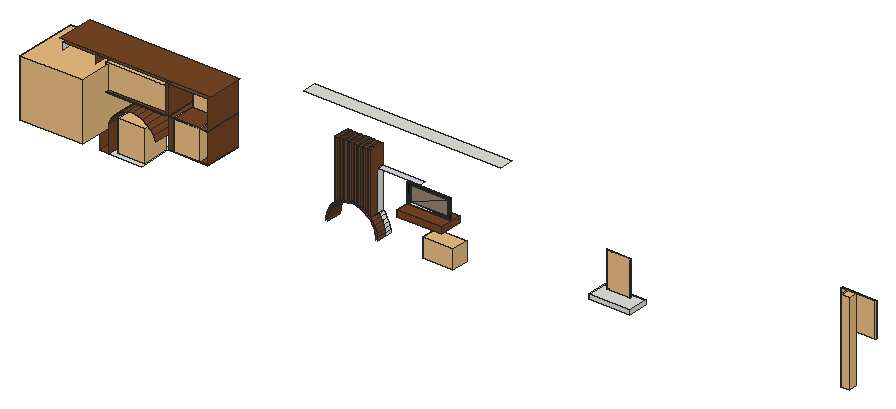
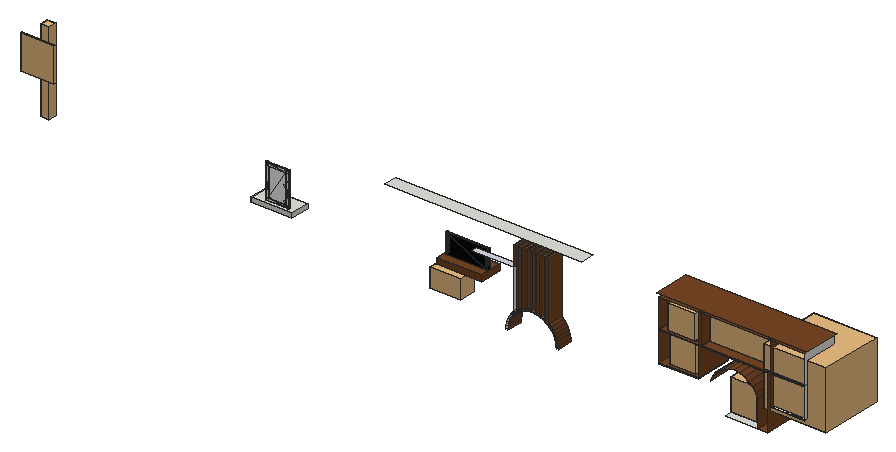
# SketchUp Ruby script. Lengths in inches.
U = 1.inch
M = Sketchup.active_model
def pt(a) = Geom::Point3d.new(a.map { |v| v * U })
def face(e, loops, mat)
  f = e.add_face(loops[0].map { |a| pt(a) })
  loops[1..].each { |l| e.add_face(l.map { |a| pt(a) }).erase! }
  f.material = f.back_material = mat if mat
  f
end
# faces: each face lists its corners as indices into pts; further lists are holes
def faces(e, pts, list, mat = nil) = list.each { |f| face(e, (f[0].is_a?(Array) ? f : [f]).map { |l| l.map { |i| pts[i] } }, mat) }
# xy, xz, yz: faces in a plane at the given z, y or x. An outline is a flat list of corners, or four numbers for a rectangle; further outlines are holes
def ring(l) = l.size == 4 ? [[l[0], l[1]], [l[2], l[1]], [l[2], l[3]], [l[0], l[3]]] : l.each_slice(2).to_a
def flat(e, list, mat, &to3) = list.each { |f| face(e, (f[0].is_a?(Array) ? f : [f]).map { |l| ring(l).map { |u, v| to3.(u, v) } }, mat) }
def xy(e, z, list, mat = nil) = flat(e, list, mat) { |x, y| [x, y, z] }
def xz(e, y, list, mat = nil) = flat(e, list, mat) { |x, z| [x, y, z] }
def yz(e, x, list, mat = nil) = flat(e, list, mat) { |y, z| [x, y, z] }
def lines(e, pts, list) = list.each { |a, b| e.add_line(pt(pts[a]), pt(pts[b])) }
# prism: a flat outline (further loops are holes) pulled along v
def prism(e, loops, v, mat = nil)
  f = face(e, loops, mat); d = Geom::Vector3d.new(v.map { |x| x * U })
  f.pushpull(f.normal.samedirection?(d) ? d.length : -d.length)
end
def box(e, o, s, mat = nil) = prism(e, [[o, [o[0] + s[0], o[1], o[2]], [o[0] + s[0], o[1] + s[1], o[2]], [o[0], o[1] + s[1], o[2]]]], [0, 0, s[2]], mat)
def at(x, y, z, deg = 0) = Geom::Transformation.translation(pt([x, y, z])) * Geom::Transformation.rotation(ORIGIN, Z_AXIS, deg.degrees)
def axes(o, x, y, z) = Geom::Transformation.new([*x, 0, *y, 0, *z, 0, *pt(o).to_a, 1])
def part(name) = M.definitions.add(name)
# library, detail: a bought-in or finely detailed component or shape, given as its bounding box
def library(name, o, s) = part(name).tap { |d| box(d.entities, o, s) }
def detail(e, o, s) = box(e.add_group.entities, o, s)
def put(e, d, t, mat = nil) = e.add_instance(d, t).tap { |i| i.material = mat if mat }
def group(e, t, mat = nil) = e.add_group.tap { |g| g.transformation = t; g.material = mat if mat }.entities
root = M.entities
M.materials.add("Material~27").color = [10, 10, 10]
M.materials.add("Material~5").color = [255, 255, 255]
M.materials.add("Material~59").color = [149, 131, 114]
M.materials.add("Material~69").color = [244, 243, 242]
M.materials.add("Material~70").color = [97, 97, 95]
M.materials.add("[Color A01]").color = [218, 217, 228]
M.materials.add("[Wood Veneer 01]").color = [120, 70, 37]
c1 = library("Potted succulent",[-1.34,0,0],[22.39,22.71,26.72])
c2 = library("Architecture and design books\#1",[9.67,-0.02,0],[20.02,11.1,12.25])
c3 = library("Potted trailing philodendron",[-13.52,-13.75,-7.41],[40.56,40.5625,37.31])
c4 = library("Livros",[0,0,0],[9.4375,8.82,3.7])
c5 = library("Untitled (9)",[-9.61,-14.59,-0.92],[76.83,66.21,110.98])
c6 = library("Ceiling Lamp 298 001",[-7.99,-7.99,-104.37],[15.97,15.98,104.68])
c7 = library("Group173\#1",[38.89,-1.29,42],[15.62,0.47,22.73])
c8 = part("3DGeom~54_Defintion\#1")
xy(c8.entities,-4.77,[[-138.48,-508.22,-215.75,-435.55,-138.48,-435.55],[-215.75,-508.22,-215.75,-435.55,-138.48,-508.22],[-138.48,-508.22,-138.48,-435.55,381.8,-435.55],[-138.48,-508.22,381.8,-435.55,381.8,-508.22],[381.8,-508.22,381.8,-435.55,453.81,-508.22],
  [453.81,-508.22,381.8,-435.55,453.81,-435.55],[-138.48,-435.55,-215.75,417.75,-138.48,417.78],[-215.75,-435.55,-215.75,417.75,-138.48,-435.55],[-138.48,-435.55,-138.48,417.78,381.8,-435.55],[381.8,-435.55,-138.48,417.78,381.8,417.78],
  [381.8,-435.55,381.8,417.78,453.81,-435.55],[453.81,-435.55,381.8,417.78,453.81,417.78],[-215.75,417.75,-215.75,491.78,-138.48,417.78],[-138.48,417.78,-215.75,491.78,-138.48,491.78],[-138.48,417.78,-138.48,491.78,381.8,491.78],
  [-138.48,417.78,381.8,491.78,381.8,417.78],[381.8,417.78,381.8,491.78,453.81,491.78],[381.8,417.78,453.81,491.78,453.81,417.78]])
xy(c8.entities,-3.49,[[-138.48,-435.55,381.8,-435.55,381.8,417.78],[-138.48,-435.55,381.8,417.78,-138.48,417.78]])
xy(c8.entities,1.08,[[-138.48,-508.22,-138.48,-435.55,-215.75,-435.55],[-215.75,-508.22,-138.48,-508.22,-215.75,-435.55],[-138.48,-508.22,381.8,-508.22,-138.48,-435.55],[381.8,-508.22,381.8,-435.55,-138.48,-435.55],[381.8,-508.22,453.81,-508.22,381.8,-435.55],
  [453.81,-508.22,453.81,-435.55,381.8,-435.55],[-215.75,-435.55,-138.48,-435.55,-138.48,417.78],[-215.75,-435.55,-138.48,417.78,-215.75,417.75],[381.8,-435.55,453.81,-435.55,453.81,417.78],[381.8,-435.55,453.81,417.78,381.8,417.78],
  [-215.75,417.75,-138.48,417.78,-138.48,491.78],[-215.75,417.75,-138.48,491.78,-215.75,491.78],[-138.48,417.78,381.8,417.78,-138.48,491.78],[381.8,417.78,381.8,491.78,-138.48,491.78],[381.8,417.78,453.81,417.78,453.81,491.78],
  [381.8,417.78,453.81,491.78,381.8,491.78]])
xz(c8.entities,-508.22,[[-138.48,-4.77,-138.48,1.08,-215.75,1.08],[-215.75,-4.77,-138.48,-4.77,-215.75,1.08],[-138.48,-4.77,381.8,-4.77,-138.48,1.08],[381.8,-4.77,381.8,1.08,-138.48,1.08],[381.8,-4.77,453.81,-4.77,381.8,1.08],
  [453.81,-4.77,453.81,1.08,381.8,1.08]])
xz(c8.entities,-435.55,[[-138.48,-3.49,-138.48,1.08,381.8,-3.49],[381.8,-3.49,-138.48,1.08,381.8,1.08]])
xz(c8.entities,417.78,[[-138.48,-3.49,381.8,-3.49,381.8,1.08],[-138.48,-3.49,381.8,1.08,-138.48,1.08]])
xz(c8.entities,491.78,[[-215.75,-4.77,-138.48,1.08,-138.48,-4.77],[-215.75,-4.77,-215.75,1.08,-138.48,1.08],[-138.48,-4.77,-138.48,1.08,381.8,1.08],[-138.48,-4.77,381.8,1.08,381.8,-4.77],[381.8,-4.77,381.8,1.08,453.81,1.08],
  [381.8,-4.77,453.81,1.08,453.81,-4.77]])
yz(c8.entities,-215.75,[[-508.22,-4.77,-435.55,1.08,-435.55,-4.77],[-508.22,-4.77,-508.22,1.08,-435.55,1.08],[-435.55,-4.77,-435.55,1.08,417.75,1.08],[-435.55,-4.77,417.75,1.08,417.75,-4.77],[417.75,-4.77,417.75,1.08,491.78,1.08],
  [417.75,-4.77,491.78,1.08,491.78,-4.77]])
yz(c8.entities,-138.48,[[-435.55,-3.49,417.78,-3.49,417.78,1.08],[-435.55,-3.49,417.78,1.08,-435.55,1.08]])
yz(c8.entities,381.8,[[-435.55,-3.49,-435.55,1.08,417.78,-3.49],[417.78,-3.49,-435.55,1.08,417.78,1.08]])
yz(c8.entities,453.81,[[-435.55,-4.77,-435.55,1.08,-508.22,1.08],[-508.22,-4.77,-435.55,-4.77,-508.22,1.08],[-435.55,-4.77,417.78,-4.77,-435.55,1.08],[417.78,-4.77,417.78,1.08,-435.55,1.08],[417.78,-4.77,491.78,-4.77,417.78,1.08],
  [491.78,-4.77,491.78,1.08,417.78,1.08]])
c9 = part("Group164\#1")
put(c9.entities,c8,axes([44.14,-0.82,53.52],[0.0216,0,0],[0,0,0.0216],[0,-0.03544,0]),"Material~69")
c10 = part("Group163\#1")
put(c10.entities,c9,at(0,0,0))
c11 = part("3DGeom~55_Defintion\#1")
xy(c11.entities,0,[[-304.85,-754.5,-304.85,-254.5,0,-254.5],[-304.85,-754.5,0,-254.5,0,-754.5],[0,-754.5,0,-254.5,304.85,-254.5],[0,-754.5,304.85,-254.5,304.85,-754.5],[-304.85,-254.5,-304.85,245.5,0,245.5],
  [-304.85,-254.5,0,245.5,0,-254.5],[0,-254.5,0,245.5,304.85,245.5],[0,-254.5,304.85,245.5,304.85,-254.5]],"Material~70")
xy(c11.entities,1.48,[[-304.85,-754.5,0,-254.5,-304.85,-254.5],[-304.85,-754.5,0,-754.5,0,-254.5],[0,-754.5,304.85,-254.5,0,-254.5],[0,-754.5,304.85,-754.5,304.85,-254.5],[-304.85,-254.5,0,-254.5,0,245.5],
  [-304.85,-254.5,0,245.5,-304.85,245.5],[0,-254.5,304.85,-254.5,304.85,245.5],[0,-254.5,304.85,245.5,0,245.5]],"Material~70")
xz(c11.entities,-754.5,[[-304.85,0,0,0,0,1.48],[-304.85,0,0,1.48,-304.85,1.48],[0,0,304.85,0,304.85,1.48],[0,0,304.85,1.48,0,1.48]],"Material~70")
xz(c11.entities,245.5,[[-304.85,0,-304.85,1.48,0,0],[0,0,-304.85,1.48,0,1.48],[0,0,0,1.48,304.85,0],[304.85,0,0,1.48,304.85,1.48]],"Material~70")
yz(c11.entities,-304.85,[[-254.5,0,-754.5,1.48,-254.5,1.48],[-754.5,0,-754.5,1.48,-254.5,0],[-254.5,0,-254.5,1.48,245.5,0],[245.5,0,-254.5,1.48,245.5,1.48]],"Material~70")
yz(c11.entities,304.85,[[-754.5,0,-254.5,0,-254.5,1.48],[-754.5,0,-254.5,1.48,-754.5,1.48],[-254.5,0,245.5,0,245.5,1.48],[-254.5,0,245.5,1.48,-254.5,1.48]],"Material~70")
c12 = part("Group166\#1")
put(c12.entities,c11,axes([46.76,-0.69,58.02],[0.01843,0,0],[0,0,0.01843],[0,-0.01843,0]),"Material~70")
c13 = part("Group165\#1")
put(c13.entities,c12,at(0,0,0))
c14 = part("3DGeom~36_Defintion")
xy(c14.entities,32.5082,[[-348.8471,305.6049,-329.3422,305.605,-329.3422,325.1098],[-348.8471,305.6049,-329.3422,325.1098,-348.847,325.1098],[-329.3422,305.605,631.6479,305.605,631.6479,325.1099],[-329.3422,305.605,631.6479,325.1099,-329.3422,325.1098],[631.6479,305.605,651.1528,305.605,651.1528,325.1098],
  [631.6479,305.605,651.1528,325.1098,631.6479,325.1099],[-329.3422,325.1098,631.6479,325.1099,651.1528,325.1098]])
xy(c14.entities,32.5084,[[-348.8471,-159.6459,-329.3422,-140.1408,-348.847,-140.1409],[-348.8471,-159.6459,-329.3422,-159.6459,-329.3422,-140.1408],[-329.3422,-159.6459,631.648,-140.1409,-329.3422,-140.1408],[-329.3422,-159.6459,631.648,-159.6458,631.648,-140.1409],[651.1529,-159.6459,651.1529,-140.1409,631.648,-159.6458],
  [631.648,-159.6458,651.1529,-140.1409,631.648,-140.1409]])
xz(c14.entities,-159.6459,[[-348.8471,0.0001,-329.3422,32.5084,-348.8471,32.5084],[-348.8471,0.0001,651.1529,0.0001,651.1529,32.5084]])
xz(c14.entities,305.605,[[-329.3422,13.0032,631.6479,32.5082,-329.3422,32.5082]])
xz(c14.entities,325.1098,[[-348.847,-0.0001,-329.3422,32.5082,651.1528,32.5082],[-348.847,-0.0001,-348.847,32.5082,-329.3422,32.5082]])
yz(c14.entities,-329.3422,[[305.605,13.0032,305.605,32.5082,-140.1409,13.0034],[-140.1409,13.0034,305.605,32.5082,-140.1408,32.5084]])
yz(c14.entities,651.1529,[[-159.6459,0.0001,-140.1409,32.5084,-159.6459,32.5084]])
p = [[-348.847,325.1098,-0.0001],[-348.8471,-159.6459,0.0001],[-348.8471,-159.6459,32.5084],[-348.847,-140.1409,32.5084],[-348.8471,-159.6459,0.0001],[651.1529,-159.6459,32.5084],
  [631.648,-159.6458,32.5084],[-329.3422,-159.6459,32.5084],[-348.8471,-159.6459,0.0001],[-348.847,325.1098,-0.0001],[651.1529,325.1099,-0.0001],[651.1529,-159.6459,0.0001],
  [651.1529,-159.6459,0.0001],[651.1529,325.1099,-0.0001],[651.1528,325.1098,32.5082],[651.1528,305.605,32.5082],[651.1529,-140.1409,32.5084],[-348.8471,305.6049,32.5082],
  [-348.847,325.1098,32.5082],[-348.847,325.1098,-0.0001],[651.1528,325.1098,32.5082],[651.1529,325.1099,-0.0001],[-329.3422,-140.1408,32.5084],[631.648,-140.1409,32.5084],
  [631.648,-140.1409,13.0034],[631.648,-140.1409,13.0034],[-329.3422,-140.1409,13.0034],[-329.3422,-140.1408,32.5084],[631.648,-140.1409,32.5084],[631.6479,305.605,32.5082],
  [631.6479,305.6049,13.0032],[631.648,-140.1409,13.0034],[-329.3422,305.605,13.0032],[631.6479,305.6049,13.0032],[631.6479,305.605,32.5082],[-329.3422,305.605,32.5082],
  [-348.8471,305.6049,32.5082],[-348.847,-140.1409,32.5084],[-329.3422,-140.1408,32.5084],[651.1529,-140.1409,32.5084],[651.1528,305.605,32.5082],[631.648,-140.1409,32.5084],
  [631.6479,305.605,32.5082]]
faces(c14.entities,p,[[0,1,2],[0,2,3],[4,5,6],[4,6,7],[8,9,10],[8,10,11],[12,13,14],[12,14,15],
  [12,15,16],[0,3,17],[0,17,18],[19,20,21],[22,23,24],[25,26,27],[28,29,30],[30,31,28],
  [32,33,34],[35,36,37],[35,37,38],[39,40,41],[41,40,42]])
c15 = part("Group132\#1")
put(c15.entities,c14,axes([19.29,-0.65,50.14],[0.0274,0,0],[0,0,0.0274],[0,-0.0274,0]),"Material~27")
c16 = part("3DGeom~37_Defintion")
xy(c16.entities,13.53,[[-342.71,-145.83,-296.47,-99.59,-342.71,318.01],[-342.71,-145.83,657.29,-145.83,-296.47,-99.59],[657.29,-145.83,611.05,-99.59,-296.47,-99.59],[657.29,-145.83,611.05,271.77,611.05,-99.59],[657.29,-145.83,657.29,318.01,611.05,271.77],
  [-296.47,-99.59,-296.47,271.77,-342.71,318.01],[-296.47,271.77,657.29,318.01,-342.71,318.01],[-296.47,271.77,611.05,271.77,657.29,318.01]])
xz(c16.entities,-99.59,[[-296.47,6.77,-296.47,13.53,611.05,6.77],[611.05,6.77,-296.47,13.53,611.05,13.53]])
xz(c16.entities,271.77,[[-296.47,6.77,611.05,13.53,-296.47,13.53],[-296.47,6.77,611.05,6.77,611.05,13.53]])
yz(c16.entities,-296.47,[[-99.59,6.77,271.77,13.53,-99.59,13.53],[-99.59,6.77,271.77,6.77,271.77,13.53]])
yz(c16.entities,611.05,[[-99.59,6.77,-99.59,13.53,271.77,6.77],[271.77,6.77,-99.59,13.53,271.77,13.53]])
c17 = part("Group133\#1")
put(c17.entities,c16,axes([19.29,-0.65,50.14],[0.02633,0,0],[0,0,0.02633],[0,-0.02633,0]),"Material~5")
c18 = part("3DGeom~38_Defintion")
p = [[673.32,299.47,7.45],[-326.68,299.47,7.45],[-326.68,-109.74,7.46],[673.32,-109.74,7.46]]
faces(c18.entities,p,[[0,1,2],[2,3,0]],"Material~59")
c19 = part("Group134\#1")
put(c19.entities,c18,axes([19.29,-0.65,50.14],[0.0239,0,0],[0,0,0.0239],[0,-0.0239,0]),"Material~59")
c20 = part("Group131\#1")
put(c20.entities,c15,at(0,0,0))
put(c20.entities,c17,at(0,0,0))
put(c20.entities,c19,at(0,0,0))
c21 = library("BOOJ",[0,0,0],[7.56,19.95,10.95])
c22 = library("Buddha-Sitting[SKU_WDMG1527]\#1",[-16.46,-2.93,-0.22],[32.92,12.37,35.44])
box(root,[344.46,13.97,98.94],[26.4,13,2.87])
box(root,[221.91,11.47,104.85],[29,15,4],"[Wood Veneer 01]")
xy(root,82.32,[[42.64,2.47,63.64,26.47]])
xy(root,82.32,[[36.38,2.47,42.64,26.47]],"[Wood Veneer 01]")
xy(root,97.89,[[12.38,2.47,34.34,26.47]])
xy(root,97.89,[[81.29,2.47,106.84,26.47]],"[Wood Veneer 01]")
xy(root,98.39,[[12.38,2.47,34.34,26.47]])
xy(root,98.39,[[81.29,2.47,106.84,26.47]],"[Wood Veneer 01]")
xy(root,98.54,[[187.93,16.47,189.89,26.47]],"[Wood Veneer 01]")
xy(root,99.93,[[188.91,16.47,189.91,26.47]],"[Wood Veneer 01]")
xy(root,117.32,[[12.38,2.47,34.34,26.47],[36.38,2.47,79.29,26.47],[81.29,2.47,81.38,26.47],[81.38,2.47,106.84,26.47]],"[Wood Veneer 01]")
xy(root,117.82,[[12.38,2.47,34.34,26.47],[36.38,2.47,79.29,26.47],[81.38,2.47,106.84,26.47]],"[Wood Veneer 01]")
xy(root,120.83,[[200.91,22.47,227.91,26.47]],"[Color A01]")
xy(root,133.83,[[177.91,16.47,179.91,26.47],[180.91,16.47,182.91,26.47],[183.91,16.47,185.91,26.47],[186.91,16.47,188.91,26.47],[189.91,16.47,191.91,26.47],
  [192.91,16.47,194.91,26.47],[195.91,16.47,197.91,26.47],[198.91,16.47,200.91,26.47]],"[Wood Veneer 01]")
xy(root,136.75,[[12.38,2.47,34.34,26.47],[34.34,2.47,36.46,26.47],[36.46,2.47,79.29,26.47],[79.29,2.47,81.29,26.47],[81.29,2.47,106.84,26.47]],"[Wood Veneer 01]")
xy(root,138.34,[[10.79,2.47,108.43,26.47]],"[Wood Veneer 01]")
xy(root,146,[[149.45,26.47,277.45,35.47]])
xz(root,2.47,[[12.38,97.89,34.34,98.39]])
xz(root,2.47,[[36.38,82.32,36.46,117.32],[81.29,97.89,106.84,98.39],[12.38,117.32,34.34,117.82],[36.38,117.32,36.46,117.82],[36.46,117.32,79.29,117.82],
  [81.38,117.32,81.46,117.82],[81.46,117.32,106.84,117.82]],"[Wood Veneer 01]")
xz(root,16.47,[[200.91,94.97,200.91,133.83,198.91,133.83,198.91,96.67,199.75,96.0625],[177.91,95.91,178.07,96.0625,179.8,97.32,179.91,97.38,179.91,133.83,177.91,133.83],[197.91,97.38,197.91,133.83,195.91,133.83,195.91,98.44,196.15,98.35],[180.91,97.93,181.67,98.35,182.91,98.84,182.91,133.83,180.91,133.83],[194.91,98.84,194.91,133.83,192.91,133.83,192.91,99.46,194.16,99.13],
  [183.91,99.2,185.72,99.66,185.91,99.6875,185.91,133.83,183.91,133.83],[191.91,99.6875,191.91,133.83,189.91,133.83,189.91,99.93,189.98,99.93],[186.91,99.8125,187.84,99.93,188.91,99.93,188.91,133.83,186.91,133.83]],"[Wood Veneer 01]")
xz(root,26.47,[[36.38,82.32,36.46,117.32],[12.38,97.89,34.34,98.39],[81.29,97.89,106.84,98.39],[12.38,117.32,34.34,117.82],[36.38,117.32,36.46,117.82],
  [36.46,117.32,79.29,117.82],[81.38,117.32,81.46,117.82],[81.46,117.32,106.84,117.82]],"[Wood Veneer 01]")
yz(root,12.38,[[2.47,98.39,26.47,117.82],[2.47,117.82,26.47,136.75]])
yz(root,34.34,[[2.47,98.39,26.47,117.82],[2.47,117.82,26.47,136.75]],"[Wood Veneer 01]")
yz(root,36.38,[[2.47,82.32,26.47,117.32],[2.47,117.32,26.47,117.82]],"[Wood Veneer 01]")
yz(root,42.64,[[2.47,82.32,26.47,99.82]],"[Wood Veneer 01]")
yz(root,79.29,[[2.47,117.32,26.47,117.82],[2.47,117.82,26.47,136.75]],"[Wood Veneer 01]")
yz(root,81.29,[[2.47,98.39,26.47,117.32],[2.47,117.32,26.47,136.75]],"[Wood Veneer 01]")
yz(root,81.38,[[2.47,117.32,26.47,117.82]],"[Wood Veneer 01]")
yz(root,106.84,[[2.47,98.39,26.47,117.32],[2.47,117.32,26.47,117.82],[2.47,117.82,26.47,136.75]],"[Wood Veneer 01]")
yz(root,177.91,[[16.47,95.91,26.47,133.83]],"[Wood Veneer 01]")
yz(root,179.91,[[16.47,97.38,26.47,133.83]],"[Wood Veneer 01]")
yz(root,180.91,[[16.47,97.93,26.47,133.83]],"[Wood Veneer 01]")
yz(root,182.91,[[16.47,98.84,26.47,133.83]],"[Wood Veneer 01]")
yz(root,183.91,[[16.47,99.2,26.47,133.83]],"[Wood Veneer 01]")
yz(root,185.91,[[16.47,99.6875,26.47,133.83]],"[Wood Veneer 01]")
yz(root,186.91,[[16.47,99.8125,26.47,133.83]],"[Wood Veneer 01]")
yz(root,188.91,[[16.47,99.93,26.47,133.83]],"[Wood Veneer 01]")
yz(root,189.91,[[16.47,99.93,26.47,133.83]],"[Wood Veneer 01]")
yz(root,191.91,[[16.47,99.6875,26.47,133.83]],"[Wood Veneer 01]")
yz(root,192.91,[[16.47,99.46,26.47,133.83]],"[Wood Veneer 01]")
yz(root,194.91,[[16.47,98.84,26.47,133.83]],"[Wood Veneer 01]")
yz(root,195.91,[[16.47,98.44,26.47,133.83]],"[Wood Veneer 01]")
yz(root,197.91,[[16.47,97.38,26.47,133.83]],"[Wood Veneer 01]")
yz(root,198.91,[[16.47,96.67,26.47,133.83]],"[Wood Veneer 01]")
yz(root,200.91,[[22.47,94.97,26.47,120.83]])
yz(root,200.91,[[16.47,94.97,22.47,94.97,22.47,120.83,26.47,120.83,26.47,133.83,16.47,133.83]],"[Wood Veneer 01]")
p = [[172.04,26.47,85.1],[171.91,26.47,82.97],[171.91,16.47,82.97],[172.04,16.47,85.1],[173.3,26.47,82.97],[173.42,26.47,84.92],
  [173.42,16.47,84.92],[173.3,16.47,82.97],[204.4,26.47,84.92],[204.52,26.47,82.97],[204.52,16.47,82.97],[204.4,16.47,84.92],
  [205.91,16.47,82.97],[205.91,22.47,82.97],[205.78,22.47,85.1],[205.78,16.47,85.1],[205.91,26.47,82.97],[205.78,26.47,85.1],
  [173.79,26.47,86.85],[173.79,16.47,86.85],[204.03,26.47,86.85],[204.03,16.47,86.85],[172.44,26.47,87.19],[172.44,16.47,87.19],
  [205.375,22.47,87.19],[205.375,16.47,87.19],[205.375,26.47,87.19],[174.4,26.47,88.71],[174.4,16.47,88.71],[203.42,26.47,88.71],
  [203.42,16.47,88.71],[173.1,26.47,89.22],[173.1,16.47,89.22],[204.72,22.47,89.22],[204.72,16.47,89.22],[204.72,26.47,89.22],
  [175.23,26.47,90.49],[175.23,16.47,90.49],[202.59,26.47,90.49],[202.59,16.47,90.49],[174.01,26.47,91.16],[174.01,16.47,91.16],
  [203.81,22.47,91.16],[203.81,16.47,91.16],[203.81,26.47,91.16],[176.28,26.47,92.14],[176.28,16.47,92.14],[201.54,26.47,92.14],
  [201.54,16.47,92.14],[175.16,26.47,92.96],[175.16,16.47,92.96],[202.66,22.47,92.96],[202.66,16.47,92.96],[202.66,26.47,92.96],
  [177.53,26.47,93.65],[177.53,16.47,93.65],[200.91,26.47,92.9],[200.29,16.47,93.65],[200.29,26.47,93.65],[176.52,26.47,94.6],
  [176.52,16.47,94.6],[201.3,22.47,94.6],[201.3,16.47,94.6],[201.3,26.47,94.6],[178.86,26.47,94.9],[178.96,26.47,94.99],
  [178.96,16.47,94.99],[178.86,16.47,94.9],[198.86,26.47,94.99],[199.96,26.47,93.96],[199.96,16.47,93.96],[198.86,16.47,94.99],
  [177.91,26.47,95.91],[177.91,16.47,95.91],[200.91,22.47,94.97],[200.91,16.47,94.97],[200.91,26.47,94.97],[180.55,26.47,96.15],
  [180.55,16.47,96.15],[197.27,26.47,96.15],[198.09,26.47,95.55],[198.09,16.47,95.55],[197.27,16.47,96.15],[180.58,26.47,96.16],
  [181.58,26.47,96.71],[182.26,26.47,97.09],[182.26,16.47,97.09],[181.58,16.47,96.71],[180.58,16.47,96.16],[195.56,26.47,97.09],
  [197.24,26.47,96.16],[197.24,16.47,96.16],[195.56,16.47,97.09],[198.91,26.47,96.67],[198.02,26.47,97.32],[198.02,16.47,97.32],
  [198.91,16.47,96.67],[183.42,26.47,97.55],[184.09,26.47,97.8125],[184.09,16.47,97.8125],[183.42,16.47,97.55],[193.73,26.47,97.8125],
  [194.4,26.47,97.55],[195.4,26.47,97.15],[195.4,16.47,97.15],[194.4,16.47,97.55],[193.73,16.47,97.8125],[197.91,26.47,97.38],
  [197.91,16.47,97.38],[180.91,26.47,97.93],[179.91,26.47,97.38],[179.91,16.47,97.38],[180.91,16.47,97.93],[184.25,26.47,97.85],
  [185.98,26.47,98.3],[185.98,16.47,98.3],[184.25,16.47,97.85],[191.83,26.47,98.3],[192.56,26.47,98.11],[192.56,16.47,98.11],
  [191.83,16.47,98.3],[186.08,26.47,98.3125],[187.08,26.47,98.4375],[187.93,26.47,98.54],[187.93,16.47,98.54],[187.08,16.47,98.4375],
  [186.08,16.47,98.3125],[189.89,26.47,98.54],[191.74,26.47,98.3125],[191.74,16.47,98.3125],[189.89,16.47,98.54],[195.91,26.47,98.44],
  [194.91,26.47,98.84],[194.91,16.47,98.84],[195.91,16.47,98.44],[183.66,26.47,99.13],[182.91,26.47,98.84],[182.91,16.47,98.84],
  [183.66,16.47,99.13],[183.91,26.47,99.2],[183.91,16.47,99.2],[192.91,26.47,99.46],[192.1,26.47,99.66],[192.1,16.47,99.66],
  [192.91,16.47,99.46],[186.91,26.47,99.8125],[185.91,26.47,99.6875],[185.91,16.47,99.6875],[186.91,16.47,99.8125],[191.91,26.47,99.6875],
  [191.91,16.47,99.6875],[43.96,2.47,102.9375],[42.64,2.47,99.82],[42.64,26.47,99.82],[43.96,26.47,102.9375],[73.11,2.47,99.82],
  [71.79,2.47,102.9375],[71.79,26.47,102.9375],[73.11,26.47,99.82],[45.9,2.47,105.7],[45.9,26.47,105.7],[69.85,2.47,105.7],
  [69.85,26.47,105.7],[48.38,2.47,108],[48.38,26.47,108],[67.36,2.47,108],[67.36,26.47,108],[51.3,2.47,109.72],
  [51.3,26.47,109.72],[64.45,2.47,109.72],[64.45,26.47,109.72],[54.51,2.47,110.78],[54.51,26.47,110.78],[61.24,2.47,110.78],
  [61.24,26.47,110.78],[57.875,2.47,111.14],[57.875,26.47,111.14]]
faces(root,p,[[0,1,2,3],[4,5,6,7],[8,9,10,11],[12,13,14,15],[5,18,19,6],[20,8,11,21],[22,0,3,23],[15,14,24,25],
  [18,27,28,19],[29,20,21,30],[31,22,23,32],[25,24,33,34],[27,36,37,28],[38,29,30,39],[40,31,32,41],[34,33,42,43],
  [36,45,46,37],[47,38,39,48],[49,40,41,50],[43,42,51,52],[45,54,55,46],[56,47,48,57,58],[59,49,50,60],[52,51,61,62],
  [54,64,65,66,67,55],[68,69,58,57,70,71],[72,59,60,73],[62,61,74,75],[65,77,78,66],[79,80,68,71,81,82],[83,84,85,86,87,88,78,77],[89,90,79,82,91,92],
  [93,94,95,96],[85,97,98,99,100,86],[101,102,103,89,92,104,105,106],[94,107,108,95],[109,110,111,112],[98,113,114,115,116,99],[117,118,101,106,119,120],[114,121,122,123,124,125,126,115],
  [127,128,117,120,129,130],[131,132,133,134],[135,136,137,138],[139,135,138,140],[141,142,143,144],[145,146,147,148],[142,149,150,143],[151,152,153,154],
  [155,156,157,158],[159,151,154,160],[156,161,162,157],[163,159,160,164],[161,165,166,162],[167,163,164,168],[165,169,170,166],[171,167,168,172],
  [169,173,174,170],[175,171,172,176],[173,175,176,174]],"[Wood Veneer 01]")
faces(root,p,[[16,17,14,13],[17,26,24,14],[26,35,33,24],[35,44,42,33],[44,53,51,42],[53,63,61,51],[63,76,74,61]])
detail(root,[493.19,32.47,127.48],[22,1,21.96])
put(root,c1,axes([47.75,4.72,83.17],[0.76,0,0],[0,0.76,0],[0,0,0.76]))
put(root,c2,at(228.88,11.47,86.65))
put(root,c3,at(13.09,-1.82,102.29))
put(root,c4,axes([14.71,12.38,98.39],[1.612,0,0],[0,1.34,0],[0,0,1]))
put(root,c5,axes([86.83,7.29,98.55],[0.21903,0,0],[0,0.33,0],[0,0,0.17508]))
put(root,c6,axes([505.14,23.69,153.94],[0.336,0,0],[0,0.3481,0],[0,0,0.5117]))
put(root,c7,at(308.93,25.26,59.82))
put(root,c10,at(308.93,25.26,59.82))
put(root,c13,at(308.93,25.26,59.82))
put(root,c20,at(212.32,21.4,62.55))
put(root,c21,axes([38.64,4.77,117.82],[0,2,0],[2.03752,0,0],[0,0,1.41]))
put(root,c22,axes([94.03,18.96,117.91],[0.5382,0,0],[0,0.58,0],[0,0,0.4425]))
